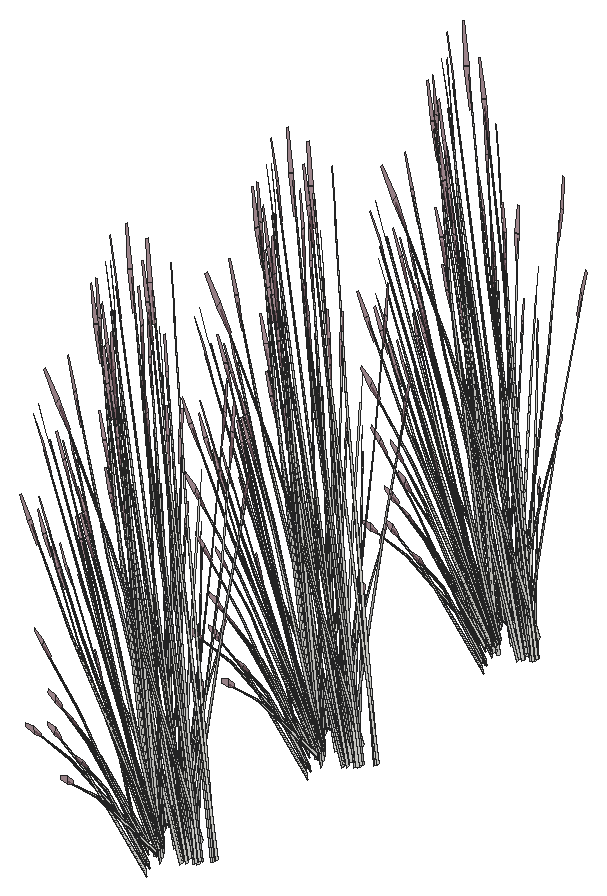
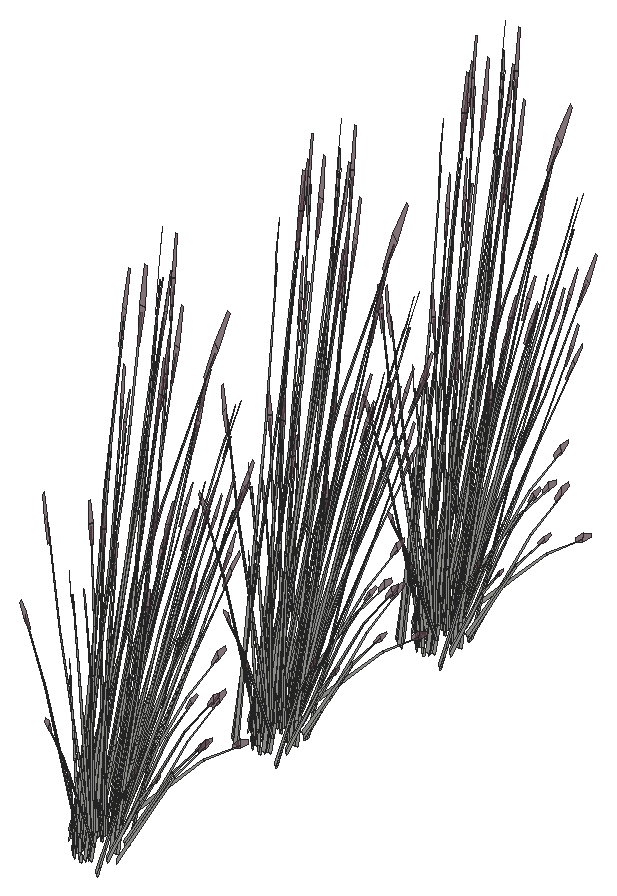
# SketchUp Ruby script. Lengths in inches.
U = 1.inch
M = Sketchup.active_model
def pt(a) = Geom::Point3d.new(a.map { |v| v * U })
def face(e, loops, mat)
  f = e.add_face(loops[0].map { |a| pt(a) })
  loops[1..].each { |l| e.add_face(l.map { |a| pt(a) }).erase! }
  f.material = f.back_material = mat if mat
  f
end
# faces: each face lists its corners as indices into pts; further lists are holes
def faces(e, pts, list, mat = nil) = list.each { |f| face(e, (f[0].is_a?(Array) ? f : [f]).map { |l| l.map { |i| pts[i] } }, mat) }
# xy, xz, yz: faces in a plane at the given z, y or x. An outline is a flat list of corners, or four numbers for a rectangle; further outlines are holes
def ring(l) = l.size == 4 ? [[l[0], l[1]], [l[2], l[1]], [l[2], l[3]], [l[0], l[3]]] : l.each_slice(2).to_a
def flat(e, list, mat, &to3) = list.each { |f| face(e, (f[0].is_a?(Array) ? f : [f]).map { |l| ring(l).map { |u, v| to3.(u, v) } }, mat) }
def xy(e, z, list, mat = nil) = flat(e, list, mat) { |x, y| [x, y, z] }
def xz(e, y, list, mat = nil) = flat(e, list, mat) { |x, z| [x, y, z] }
def yz(e, x, list, mat = nil) = flat(e, list, mat) { |y, z| [x, y, z] }
def lines(e, pts, list) = list.each { |a, b| e.add_line(pt(pts[a]), pt(pts[b])) }
# prism: a flat outline (further loops are holes) pulled along v
def prism(e, loops, v, mat = nil)
  f = face(e, loops, mat); d = Geom::Vector3d.new(v.map { |x| x * U })
  f.pushpull(f.normal.samedirection?(d) ? d.length : -d.length)
end
def box(e, o, s, mat = nil) = prism(e, [[o, [o[0] + s[0], o[1], o[2]], [o[0] + s[0], o[1] + s[1], o[2]], [o[0], o[1] + s[1], o[2]]]], [0, 0, s[2]], mat)
def at(x, y, z, deg = 0) = Geom::Transformation.translation(pt([x, y, z])) * Geom::Transformation.rotation(ORIGIN, Z_AXIS, deg.degrees)
def axes(o, x, y, z) = Geom::Transformation.new([*x, 0, *y, 0, *z, 0, *pt(o).to_a, 1])
def part(name) = M.definitions.add(name)
# library, detail: a bought-in or finely detailed component or shape, given as its bounding box
def library(name, o, s) = part(name).tap { |d| box(d.entities, o, s) }
def detail(e, o, s) = box(e.add_group.entities, o, s)
def put(e, d, t, mat = nil) = e.add_instance(d, t).tap { |i| i.material = mat if mat }
def group(e, t, mat = nil) = e.add_group.tap { |g| g.transformation = t; g.material = mat if mat }.entities
root = M.entities
M.materials.add("LightPink_Translucent").color = [144, 107, 117]
M.materials["LightPink_Translucent"].alpha = 0.75
c1 = part("blade")
p = [[2.15,0.21,22],[0,0.17,0],[0.09,0.45,0],[2.18,0.31,22],[2.29,0.31,22],[0.38,0.45,0],
  [2.48,0.24,33],[2.49,0.24,33],[2.48,0.22,33]]
faces(c1.entities,p,[[0,1,2,3],[4,5,2,3],[6,3,4,7],[8,0,3,6]])
c2 = part("seeds")
p = [[0.3,-0.1,1.38],[-0.01,-0.03,1.59],[-0.01,-0.03,0.03],[0.14,-0.07,-0.07],[0.29,-0.03,3],[0.15,0.01,3.11]]
faces(c2.entities,p,[[0,1,2,3],[1,0,4,5]],"LightPink_Translucent")
c3 = part("blade with seeds")
put(c3.entities,c1,at(0,0,0))
put(c3.entities,c2,axes([2.4,0.25,30.99],[1.5799,-0.05474,1.17369],[-0.12525,1.92788,0.29478],[-0.07173,-0.02425,1.56792]))
put(root,c3,axes([505.72,495.22,3.91],[-0.11621,-0.08567,1.74944],[-0.77555,0.05431,-0.27667],[-0.12378,-0.20491,0.14031]))
put(root,c3,axes([504.18,496,1.78],[-0.04601,0.19989,1.43002],[-0.67263,0.16733,-0.30754],[-0.15723,-0.25836,0.61141]))
put(root,c3,axes([504.93,494.94,3.9],[-0.01417,0.07324,1.77383],[-0.6991,0.2658,-0.16761],[-0.20573,-0.13587,0.31391]))
put(root,c3,axes([504.77,496.24,4.29],[0.84639,-0.15705,0.53763],[0.14689,0.61608,0.4433],[-0.19906,-0.18157,1.11249]))
put(root,c3,axes([503.95,495.68,1.96],[0.39634,0.21267,1.1486],[-0.57721,0.12784,0.84392],[-0.1235,-0.16344,0.25299]))
put(root,c3,axes([504.9,496.81,4.17],[-0.64788,-0.29534,-0.71045],[0.46044,-0.51755,0.08574],[-0.23473,-0.17635,1.00501]))
put(root,c3,axes([504.68,496.42,3.72],[-0.11735,-0.49217,-0.35414],[0.67083,-0.12996,0.4572],[-0.18018,-0.14104,0.87481]))
put(root,c3,axes([504.97,496.37,3.92],[0.34533,-0.38816,0.0643],[0.49176,0.22599,0.50621],[-0.15898,-0.12445,0.77189]))
put(root,c3,axes([503.63,496.32,0.6875],[-0.0736,0.08049,1.76342],[-0.74378,0.17355,-0.26939],[-0.17968,-0.15788,0.30037]))
put(root,c3,axes([504.6,496.82,3.875],[-0.74975,0.14525,-0.51099],[-0.13115,-0.55007,-0.3958],[-0.20138,-0.15763,0.97773]))
put(root,c3,axes([505.125,496.33,4.62],[-0.50709,0.58578,-0.13619],[-0.73436,-0.33748,-0.75594],[-0.25527,-0.1655,1.14864]))
put(root,c3,axes([503.18,496.16,3.91],[-0.16348,-0.00431,1.74944],[-0.52047,0.43131,-0.27667],[-0.2777,-0.08813,0.14031]))
put(root,c3,axes([506.45,500.15,2.52],[0.65659,0.2464,1.51261],[-0.64324,0.53082,0.59816],[-0.28812,-0.31461,1.26806]))
put(root,c3,axes([505.08,496.82,4.24],[0.11735,0.49217,0.35414],[-0.67083,0.12996,-0.4572],[-0.18018,-0.14104,0.87481]))
put(root,c3,axes([503.02,498.45,1.21],[0,-0.61104,-0.49651],[0.85008,0,0],[0,-0.13917,1.57504]))
put(root,c3,axes([503.0625,497.14,4.29],[0.62747,-0.45094,0.53763],[0.54116,0.47889,0.4433],[-0.29439,-0.08318,1.11249]))
put(root,c3,axes([503.35,497.14,3.92],[0.03826,-0.46465,0.0643],[0.57772,0.01274,0.50621],[-0.2213,-0.04862,0.77189]))
put(root,c3,axes([503.125,497.28,3.72],[-0.43232,-0.38257,-0.35414],[0.49364,-0.36215,0.4572],[-0.25081,-0.0551,0.87481]))
put(root,c3,axes([503.17,496.63,1.32],[-0.21918,0.49894,-0.03893],[-0.6746,-0.15348,-0.17649],[-0.10242,-0.08161,0.58215]))
put(root,c3,axes([502.81,498.91,1.57],[-0.95008,0,0],[0,-0.68292,-0.51607],[0,-0.15554,1.63711]))
put(root,c3,axes([503.54,498.73,1.52],[-0.70674,0.51372,0.30756],[-0.70717,-0.50832,-0.36492],[-0.02468,-0.14589,1.64885]))
put(root,c3,axes([505.46,499.8,1.63],[0.20138,-0.72405,-0.23429],[0.95485,0.12621,0.51271],[-0.16685,-0.09999,1.5644]))
put(root,c3,axes([503.74,497.48,4.24],[0.43232,0.38257,0.35414],[-0.49364,0.36215,-0.4572],[-0.25081,-0.0551,0.87481]))
put(root,c3,axes([502.09,498.2,1.96],[0.48508,-0.04372,1.1486],[-0.3077,0.38525,0.84392],[-0.23971,-0.05779,0.25299]))
put(root,c3,axes([503.62,497.24,4.23],[-0.04068,0.62141,-0.1216],[-0.77029,-0.01698,-0.67495],[-0.29667,-0.04317,1.02557]))
put(root,c3,axes([503.38,499.01,1.67],[0,0.61104,0.49651],[-0.85008,0,0],[0,-0.13917,1.57504]))
put(root,c3,axes([505.39,499.51,1.4],[-0.45644,-0.51287,-0.44739],[0.69137,-0.36116,0.21531],[-0.14771,-0.06346,1.43643]))
put(root,c3,axes([504.98,499.7,1.25],[-0.79037,-0.10018,-0.62353],[0.16679,-0.61794,-0.16365],[-0.23587,-0.07488,1.37633]))
put(root,c3,axes([502.51,498.55,3.93],[0.21466,-0.55714,0.48003],[0.70573,0.19051,0.3958],[-0.27753,0.03348,0.9933]))
put(root,c3,axes([502.46,498.4,3.92],[-0.27906,-0.41663,0.0643],[0.50888,-0.20393,0.50621],[-0.22432,0.04024,0.77189]))
put(root,c3,axes([504.14,500.64,1.22],[-0.17848,-0.53243,-0.30978],[0.70886,-0.15119,0.30978],[-0.1429,-0.0614,1.38974]))
put(root,c3,axes([503.94,500.87,1.21],[-0.7111,-0.30552,-0.49651],[0.42504,-0.54784,0],[-0.16196,-0.06958,1.57504]))
put(root,c3,axes([505.88,499.79,1.86],[-0.76714,0.40567,-0.29095],[-0.51013,-0.57321,-0.50002],[-0.18927,-0.05821,1.59708]))
put(root,c3,axes([505.81,499.97,1.81],[-0.14658,0.54532,0.1448],[-0.71613,-0.09466,-0.41347],[-0.13033,-0.05599,1.26744]))
put(root,c3,axes([503.03,498.56,4.24],[0.63144,0.17046,0.35414],[-0.18417,0.49731,-0.4572],[-0.25423,0.0456,0.87481]))
put(root,c3,axes([506.74,499.98,1.66],[-0.74193,-0.49181,-0.25192],[0.6243,-0.55226,0.5513],[-0.19979,0.05753,1.68216]))
put(root,c3,axes([504.79,500.92,1.67],[0.7111,0.30552,0.49651],[-0.42504,0.54784,0],[-0.16196,-0.06958,1.57504]))
put(root,c3,axes([502.76,498.39,4.23],[0.38229,0.5533,-0.1216],[-0.6785,0.2719,-0.67495],[-0.28593,0.073,1.02557]))
put(root,c3,axes([504.38,501.24,1.57],[-0.47504,0.61229,0],[-0.79476,-0.34146,-0.51607],[-0.18101,-0.07777,1.63711]))
put(root,c3,axes([506.36,499.875,1.4],[-0.82508,0.03772,-0.44739],[-0.07462,-0.62614,0.21531],[-0.14771,0.06346,1.43643]))
put(root,c3,axes([507.28,501.33,1.39],[-0.46912,-0.61443,-0.05142],[0.79476,-0.34146,0.51607],[-0.19584,0.0585,1.6363]))
put(root,c3,axes([502.68,499.9375,3.93],[-0.18844,-0.56237,0.48003],[0.73919,-0.0976,0.3958],[-0.21785,0.13226,0.9933]))
put(root,c3,axes([502.53,499.83,3.92],[-0.52161,-0.25698,0.0643],[0.30368,-0.36595,0.50621],[-0.16723,0.11831,0.77189]))
put(root,c3,axes([507.0625,501.25,1.22],[-0.70886,-0.15119,-0.30978],[0.17848,-0.53243,0.30978],[-0.1429,0.0614,1.38974]))
put(root,c3,axes([503.13,499.75,4.24],[0.66138,-0.08733,0.35414],[0.17464,0.49921,-0.4572],[-0.18953,0.13408,0.87481]))
put(root,c3,axes([501.4,501.24,1.96],[0.31665,-0.27694,1.1486],[0.12495,0.43841,0.84392],[-0.22883,0.0785,0.25299]))
put(root,c3,axes([502.59,500.05,3.72],[-0.66138,0.08733,-0.35414],[-0.17464,-0.49921,0.4572],[-0.18953,0.13408,0.87481]))
put(root,c3,axes([501.63,501.17,4.84],[0.67048,0.16311,-0.06488],[-0.20625,0.50201,-0.29416],[-0.10966,0.07622,0.97024]))
put(root,c3,axes([506.39,500.24,1.25],[-0.51177,0.45928,-0.62353],[-0.63575,-0.41646,-0.16365],[-0.20507,0.11457,1.37633]))
put(root,c3,axes([507.23,501.49,1.21],[-0.7111,0.30552,-0.49651],[-0.42504,-0.54784,0],[-0.16196,0.06958,1.57504]))
put(root,c3,axes([502.79,499.7,4.23],[0.70283,0.33692,-0.1216],[-0.40491,0.48793,-0.67495],[-0.19857,0.16961,1.02557]))
put(root,c3,axes([503.74,499.55,3.07],[0.18977,-0.18775,1.71376],[0.47917,0.50677,0.13857],[-0.32866,0.23079,0.73262]))
put(root,c3,axes([503.14,500.1,3.875],[0.19519,0.55794,-0.51099],[-0.73919,0.0976,-0.3958],[-0.21183,0.14986,0.97773]))
put(root,c3,axes([503.56,501.04,3.92],[-0.62439,-0.02847,0.0643],[0.01712,-0.42991,0.50621],[-0.06534,0.16468,0.77189]))
put(root,c3,axes([502.23,501.53,0.6875],[0.10192,0.06105,1.76342],[0.17281,0.56562,-0.26939],[-0.22588,0.12062,0.30037]))
put(root,c3,axes([503.76,501.08,3.93],[-0.54105,-0.41691,0.48003],[0.57458,-0.35956,0.3958],[-0.0998,0.1956,0.9933]))
put(root,c3,axes([503.59,500.02,3.07],[0.14147,-0.21002,1.71376],[0.59349,0.43464,0.13857],[-0.26773,0.27089,0.73262]))
put(root,c3,axes([503.76,501.2,3.72],[-0.5141,0.32171,-0.35414],[-0.48666,-0.36734,0.4572],[-0.07405,0.18664,0.87481]))
put(root,c3,axes([501.98,501.11,3.91],[-0.01889,0.12092,1.74944],[0.53598,0.42065,-0.27667],[-0.14032,0.19892,0.14031]))
put(root,c3,axes([504.08,502.45,1.96],[-0.01966,-0.36332,1.1486],[0.49135,0.25914,0.84392],[-0.09663,0.17317,0.25299]))
put(root,c3,axes([504.27,501.05,4.2],[0.54391,0.41056,-0.5672],[-0.57458,0.35956,-0.43934],[-0.08276,0.2086,1.08528]))
put(root,c3,axes([504.1,500.86,4.53],[-0.01977,0.56521,-0.7886],[-0.83252,-0.03796,0.09517],[-0.08786,0.23945,1.11556]))
put(root,c3,axes([501.92,502.35,3.9],[0.0862,-0.03689,1.77383],[0.71245,0.24539,-0.16761],[-0.01674,0.20431,0.31391]))
put(root,c3,axes([503.51,502.13,1.78],[0.23977,-0.09639,1.43002],[0.59198,0.29065,-0.30754],[-0.1762,0.25149,0.61141]))
put(root,c3,axes([503.82,501.66,2.56],[0.01669,-0.31544,1.54345],[0.75083,0.16661,0.21329],[-0.06506,0.33618,0.72882]))
put(root,c3,axes([504.63,518.62,3.07],[0.17368,0.19618,1.71376],[-0.80256,0.16516,0.13857],[-0.18139,-0.30799,0.73262]))
put(root,c3,axes([505.96,517.32,3.91],[-0.11621,-0.08567,1.74944],[-0.77555,0.05431,-0.27667],[-0.12378,-0.20491,0.14031]))
put(root,c3,axes([504.41,518.1,1.78],[-0.04601,0.19989,1.43002],[-0.67263,0.16733,-0.30754],[-0.15723,-0.25836,0.61141]))
put(root,c3,axes([505.16,517.04,3.9],[-0.01417,0.07324,1.77383],[-0.6991,0.2658,-0.16761],[-0.20573,-0.13587,0.31391]))
put(root,c3,axes([505.01,518.34,4.29],[0.84639,-0.15705,0.53763],[0.14689,0.61608,0.4433],[-0.19906,-0.18157,1.11249]))
put(root,c3,axes([504.18,517.78,1.96],[0.39634,0.21267,1.1486],[-0.57721,0.12784,0.84392],[-0.1235,-0.16344,0.25299]))
put(root,c3,axes([505.14,518.91,4.17],[-0.64788,-0.29534,-0.71045],[0.46044,-0.51755,0.08574],[-0.23473,-0.17635,1.00501]))
put(root,c3,axes([504.91,518.52,3.72],[-0.11735,-0.49217,-0.35414],[0.67083,-0.12996,0.4572],[-0.18018,-0.14104,0.87481]))
put(root,c3,axes([505.2,518.47,3.92],[0.34533,-0.38816,0.0643],[0.49176,0.22599,0.50621],[-0.15898,-0.12445,0.77189]))
put(root,c3,axes([503.87,518.42,0.6875],[-0.0736,0.08049,1.76342],[-0.74378,0.17355,-0.26939],[-0.17968,-0.15788,0.30037]))
put(root,c3,axes([504.83,518.92,3.875],[-0.74975,0.14525,-0.51099],[-0.13115,-0.55007,-0.3958],[-0.20138,-0.15763,0.97773]))
put(root,c3,axes([505.36,518.43,4.62],[-0.50709,0.58578,-0.13619],[-0.73436,-0.33748,-0.75594],[-0.25527,-0.1655,1.14864]))
put(root,c3,axes([503.41,518.26,3.91],[-0.16348,-0.00431,1.74944],[-0.52047,0.43131,-0.27667],[-0.2777,-0.08813,0.14031]))
put(root,c3,axes([506.6875,522.25,2.52],[0.65659,0.2464,1.51261],[-0.64324,0.53082,0.59816],[-0.28812,-0.31461,1.26806]))
put(root,c3,axes([505.31,518.92,4.24],[0.11735,0.49217,0.35414],[-0.67083,0.12996,-0.4572],[-0.18018,-0.14104,0.87481]))
put(root,c3,axes([503.25,520.54,1.21],[0,-0.61104,-0.49651],[0.85008,0,0],[0,-0.13917,1.57504]))
put(root,c3,axes([503.29,519.24,4.29],[0.62747,-0.45094,0.53763],[0.54116,0.47889,0.4433],[-0.29439,-0.08318,1.11249]))
put(root,c3,axes([503.58,519.23,3.92],[0.03826,-0.46465,0.0643],[0.57772,0.01274,0.50621],[-0.2213,-0.04862,0.77189]))
put(root,c3,axes([503.36,519.38,3.72],[-0.43232,-0.38257,-0.35414],[0.49364,-0.36215,0.4572],[-0.25081,-0.0551,0.87481]))
put(root,c3,axes([503.4,518.73,1.32],[-0.21918,0.49894,-0.03893],[-0.6746,-0.15348,-0.17649],[-0.10242,-0.08161,0.58215]))
put(root,c3,axes([503.04,521.01,1.57],[-0.95008,0,0],[0,-0.68292,-0.51607],[0,-0.15554,1.63711]))
put(root,c3,axes([503.78,520.83,1.52],[-0.70674,0.51372,0.30756],[-0.70717,-0.50832,-0.36492],[-0.02468,-0.14589,1.64885]))
put(root,c3,axes([502.79,518.63,3.9],[0.05633,0.06098,1.77383],[-0.27155,0.54815,-0.16761],[-0.27501,0.00397,0.31391]))
put(root,c3,axes([505.69,521.9,1.63],[0.20138,-0.72405,-0.23429],[0.95485,0.12621,0.51271],[-0.16685,-0.09999,1.5644]))
put(root,c3,axes([503.97,519.58,4.24],[0.43232,0.38257,0.35414],[-0.49364,0.36215,-0.4572],[-0.25081,-0.0551,0.87481]))
put(root,c3,axes([502.32,520.3,1.96],[0.48508,-0.04372,1.1486],[-0.3077,0.38525,0.84392],[-0.23971,-0.05779,0.25299]))
put(root,c3,axes([503.85,519.34,4.23],[-0.04068,0.62141,-0.1216],[-0.77029,-0.01698,-0.67495],[-0.29667,-0.04317,1.02557]))
put(root,c3,axes([503.62,521.11,1.67],[0,0.61104,0.49651],[-0.85008,0,0],[0,-0.13917,1.57504]))
put(root,c3,axes([505.625,521.6,1.4],[-0.45644,-0.51287,-0.44739],[0.69137,-0.36116,0.21531],[-0.14771,-0.06346,1.43643]))
put(root,c3,axes([505.22,521.8,1.25],[-0.79037,-0.10018,-0.62353],[0.16679,-0.61794,-0.16365],[-0.23587,-0.07488,1.37633]))
put(root,c3,axes([502.74,520.65,3.93],[0.21466,-0.55714,0.48003],[0.70573,0.19051,0.3958],[-0.27753,0.03348,0.9933]))
put(root,c3,axes([502.6875,520.5,3.92],[-0.27906,-0.41663,0.0643],[0.50888,-0.20393,0.50621],[-0.22432,0.04024,0.77189]))
put(root,c3,axes([504.375,522.74,1.22],[-0.17848,-0.53243,-0.30978],[0.70886,-0.15119,0.30978],[-0.1429,-0.0614,1.38974]))
put(root,c3,axes([504.18,522.97,1.21],[-0.7111,-0.30552,-0.49651],[0.42504,-0.54784,0],[-0.16196,-0.06958,1.57504]))
put(root,c3,axes([506.11,521.89,1.86],[-0.76714,0.40567,-0.29095],[-0.51013,-0.57321,-0.50002],[-0.18927,-0.05821,1.59708]))
put(root,c3,axes([506.04,522.07,1.81],[-0.14658,0.54532,0.1448],[-0.71613,-0.09466,-0.41347],[-0.13033,-0.05599,1.26744]))
put(root,c3,axes([503.26,520.65,4.24],[0.63144,0.17046,0.35414],[-0.18417,0.49731,-0.4572],[-0.25423,0.0456,0.87481]))
put(root,c3,axes([506.97,522.08,1.66],[-0.74193,-0.49181,-0.25192],[0.6243,-0.55226,0.5513],[-0.19979,0.05753,1.68216]))
put(root,c3,axes([505.02,523.02,1.67],[0.7111,0.30552,0.49651],[-0.42504,0.54784,0],[-0.16196,-0.06958,1.57504]))
put(root,c3,axes([503,520.49,4.23],[0.38229,0.5533,-0.1216],[-0.6785,0.2719,-0.67495],[-0.28593,0.073,1.02557]))
put(root,c3,axes([504.61,523.34,1.57],[-0.47504,0.61229,0],[-0.79476,-0.34146,-0.51607],[-0.18101,-0.07777,1.63711]))
put(root,c3,axes([506.6,521.97,1.4],[-0.82508,0.03772,-0.44739],[-0.07462,-0.62614,0.21531],[-0.14771,0.06346,1.43643]))
put(root,c3,axes([507.51,523.42,1.39],[-0.46912,-0.61443,-0.05142],[0.79476,-0.34146,0.51607],[-0.19584,0.0585,1.6363]))
put(root,c3,axes([502.91,522.03,3.93],[-0.18844,-0.56237,0.48003],[0.73919,-0.0976,0.3958],[-0.21785,0.13226,0.9933]))
put(root,c3,axes([502.77,521.93,3.92],[-0.52161,-0.25698,0.0643],[0.30368,-0.36595,0.50621],[-0.16723,0.11831,0.77189]))
put(root,c3,axes([503.37,521.85,4.24],[0.66138,-0.08733,0.35414],[0.17464,0.49921,-0.4572],[-0.18953,0.13408,0.87481]))
put(root,c3,axes([501.63,523.34,1.96],[0.31665,-0.27694,1.1486],[0.12495,0.43841,0.84392],[-0.22883,0.0785,0.25299]))
put(root,c3,axes([502.83,522.14,3.72],[-0.66138,0.08733,-0.35414],[-0.17464,-0.49921,0.4572],[-0.18953,0.13408,0.87481]))
put(root,c3,axes([501.87,523.26,4.84],[0.67048,0.16311,-0.06488],[-0.20625,0.50201,-0.29416],[-0.10966,0.07622,0.97024]))
put(root,c3,axes([506.62,522.33,1.25],[-0.51177,0.45928,-0.62353],[-0.63575,-0.41646,-0.16365],[-0.20507,0.11457,1.37633]))
put(root,c3,axes([507.46,523.59,1.21],[-0.7111,0.30552,-0.49651],[-0.42504,-0.54784,0],[-0.16196,0.06958,1.57504]))
put(root,c3,axes([503.02,521.8,4.23],[0.70283,0.33692,-0.1216],[-0.40491,0.48793,-0.67495],[-0.19857,0.16961,1.02557]))
put(root,c3,axes([503.97,521.65,3.07],[0.18977,-0.18775,1.71376],[0.47917,0.50677,0.13857],[-0.32866,0.23079,0.73262]))
put(root,c3,axes([503.37,522.2,3.875],[0.19519,0.55794,-0.51099],[-0.73919,0.0976,-0.3958],[-0.21183,0.14986,0.97773]))
put(root,c3,axes([503.79,523.13,3.92],[-0.62439,-0.02847,0.0643],[0.01712,-0.42991,0.50621],[-0.06534,0.16468,0.77189]))
put(root,c3,axes([502.47,523.625,0.6875],[0.10192,0.06105,1.76342],[0.17281,0.56562,-0.26939],[-0.22588,0.12062,0.30037]))
put(root,c3,axes([503.99,523.17,3.93],[-0.54105,-0.41691,0.48003],[0.57458,-0.35956,0.3958],[-0.0998,0.1956,0.9933]))
put(root,c3,axes([503.83,522.11,3.07],[0.14147,-0.21002,1.71376],[0.59349,0.43464,0.13857],[-0.26773,0.27089,0.73262]))
put(root,c3,axes([503.99,523.3,3.72],[-0.5141,0.32171,-0.35414],[-0.48666,-0.36734,0.4572],[-0.07405,0.18664,0.87481]))
put(root,c3,axes([502.22,523.2,3.91],[-0.01889,0.12092,1.74944],[0.53598,0.42065,-0.27667],[-0.14032,0.19892,0.14031]))
put(root,c3,axes([504.32,524.55,1.96],[-0.01966,-0.36332,1.1486],[0.49135,0.25914,0.84392],[-0.09663,0.17317,0.25299]))
put(root,c3,axes([504.33,522.96,4.53],[-0.01977,0.56521,-0.7886],[-0.83252,-0.03796,0.09517],[-0.08786,0.23945,1.11556]))
put(root,c3,axes([502.16,524.44,3.9],[0.0862,-0.03689,1.77383],[0.71245,0.24539,-0.16761],[-0.01674,0.20431,0.31391]))
put(root,c3,axes([503.75,524.23,1.78],[0.23977,-0.09639,1.43002],[0.59198,0.29065,-0.30754],[-0.1762,0.25149,0.61141]))
put(root,c3,axes([504.06,523.75,2.56],[0.01669,-0.31544,1.54345],[0.75083,0.16661,0.21329],[-0.06506,0.33618,0.72882]))
put(root,c3,axes([504.76,542.87,3.07],[0.17368,0.19618,1.71376],[-0.80256,0.16516,0.13857],[-0.18139,-0.30799,0.73262]))
put(root,c3,axes([504.54,542.35,1.78],[-0.04601,0.19989,1.43002],[-0.67263,0.16733,-0.30754],[-0.15723,-0.25836,0.61141]))
put(root,c3,axes([505.29,541.29,3.9],[-0.01417,0.07324,1.77383],[-0.6991,0.2658,-0.16761],[-0.20573,-0.13587,0.31391]))
put(root,c3,axes([505.14,542.59,4.29],[0.84639,-0.15705,0.53763],[0.14689,0.61608,0.4433],[-0.19906,-0.18157,1.11249]))
put(root,c3,axes([504.3125,542.03,1.96],[0.39634,0.21267,1.1486],[-0.57721,0.12784,0.84392],[-0.1235,-0.16344,0.25299]))
put(root,c3,axes([505.27,543.16,4.17],[-0.64788,-0.29534,-0.71045],[0.46044,-0.51755,0.08574],[-0.23473,-0.17635,1.00501]))
put(root,c3,axes([505.04,542.77,3.72],[-0.11735,-0.49217,-0.35414],[0.67083,-0.12996,0.4572],[-0.18018,-0.14104,0.87481]))
put(root,c3,axes([505.33,542.72,3.92],[0.34533,-0.38816,0.0643],[0.49176,0.22599,0.50621],[-0.15898,-0.12445,0.77189]))
put(root,c3,axes([504,542.67,0.6875],[-0.0736,0.08049,1.76342],[-0.74378,0.17355,-0.26939],[-0.17968,-0.15788,0.30037]))
put(root,c3,axes([504.96,543.17,3.875],[-0.74975,0.14525,-0.51099],[-0.13115,-0.55007,-0.3958],[-0.20138,-0.15763,0.97773]))
put(root,c3,axes([505.49,542.68,4.62],[-0.50709,0.58578,-0.13619],[-0.73436,-0.33748,-0.75594],[-0.25527,-0.1655,1.14864]))
put(root,c3,axes([503.54,542.51,3.91],[-0.16348,-0.00431,1.74944],[-0.52047,0.43131,-0.27667],[-0.2777,-0.08813,0.14031]))
put(root,c3,axes([506.82,546.5,2.52],[0.65659,0.2464,1.51261],[-0.64324,0.53082,0.59816],[-0.28812,-0.31461,1.26806]))
put(root,c3,axes([505.44,543.17,4.24],[0.11735,0.49217,0.35414],[-0.67083,0.12996,-0.4572],[-0.18018,-0.14104,0.87481]))
put(root,c3,axes([503.42,543.49,4.29],[0.62747,-0.45094,0.53763],[0.54116,0.47889,0.4433],[-0.29439,-0.08318,1.11249]))
put(root,c3,axes([503.71,543.49,3.92],[0.03826,-0.46465,0.0643],[0.57772,0.01274,0.50621],[-0.2213,-0.04862,0.77189]))
put(root,c3,axes([503.49,543.63,3.72],[-0.43232,-0.38257,-0.35414],[0.49364,-0.36215,0.4572],[-0.25081,-0.0551,0.87481]))
put(root,c3,axes([503.53,542.98,1.32],[-0.21918,0.49894,-0.03893],[-0.6746,-0.15348,-0.17649],[-0.10242,-0.08161,0.58215]))
put(root,c3,axes([503.17,545.26,1.57],[-0.95008,0,0],[0,-0.68292,-0.51607],[0,-0.15554,1.63711]))
put(root,c3,axes([503.91,545.08,1.52],[-0.70674,0.51372,0.30756],[-0.70717,-0.50832,-0.36492],[-0.02468,-0.14589,1.64885]))
put(root,c3,axes([502.92,542.88,3.9],[0.05633,0.06098,1.77383],[-0.27155,0.54815,-0.16761],[-0.27501,0.00397,0.31391]))
put(root,c3,axes([505.82,546.15,1.63],[0.20138,-0.72405,-0.23429],[0.95485,0.12621,0.51271],[-0.16685,-0.09999,1.5644]))
put(root,c3,axes([503.69,544.01,3.875],[-0.55171,0.40476,-0.51099],[-0.48318,-0.42758,-0.3958],[-0.28031,-0.06159,0.97773]))
put(root,c3,axes([504.1,543.83,4.24],[0.43232,0.38257,0.35414],[-0.49364,0.36215,-0.4572],[-0.25081,-0.0551,0.87481]))
put(root,c3,axes([502.45,544.55,1.96],[0.48508,-0.04372,1.1486],[-0.3077,0.38525,0.84392],[-0.23971,-0.05779,0.25299]))
put(root,c3,axes([503.98,543.59,4.23],[-0.04068,0.62141,-0.1216],[-0.77029,-0.01698,-0.67495],[-0.29667,-0.04317,1.02557]))
put(root,c3,axes([505.76,545.86,1.4],[-0.45644,-0.51287,-0.44739],[0.69137,-0.36116,0.21531],[-0.14771,-0.06346,1.43643]))
put(root,c3,axes([505.35,546.05,1.25],[-0.79037,-0.10018,-0.62353],[0.16679,-0.61794,-0.16365],[-0.23587,-0.07488,1.37633]))
put(root,c3,axes([502.875,544.9,3.93],[0.21466,-0.55714,0.48003],[0.70573,0.19051,0.3958],[-0.27753,0.03348,0.9933]))
put(root,c3,axes([502.82,544.75,3.92],[-0.27906,-0.41663,0.0643],[0.50888,-0.20393,0.50621],[-0.22432,0.04024,0.77189]))
put(root,c3,axes([502.81,545.18,0.6875],[0.01927,0.0963,1.76342],[-0.38846,0.5029,-0.26939],[-0.27592,-0.02535,0.30037]))
put(root,c3,axes([504.51,546.99,1.22],[-0.17848,-0.53243,-0.30978],[0.70886,-0.15119,0.30978],[-0.1429,-0.0614,1.38974]))
put(root,c3,axes([504.31,547.22,1.21],[-0.7111,-0.30552,-0.49651],[0.42504,-0.54784,0],[-0.16196,-0.06958,1.57504]))
put(root,c3,axes([506.24,546.14,1.86],[-0.76714,0.40567,-0.29095],[-0.51013,-0.57321,-0.50002],[-0.18927,-0.05821,1.59708]))
put(root,c3,axes([506.17,546.32,1.81],[-0.14658,0.54532,0.1448],[-0.71613,-0.09466,-0.41347],[-0.13033,-0.05599,1.26744]))
put(root,c3,axes([503.39,544.91,4.24],[0.63144,0.17046,0.35414],[-0.18417,0.49731,-0.4572],[-0.25423,0.0456,0.87481]))
put(root,c3,axes([507.1,546.33,1.66],[-0.74193,-0.49181,-0.25192],[0.6243,-0.55226,0.5513],[-0.19979,0.05753,1.68216]))
put(root,c3,axes([505.15,547.27,1.67],[0.7111,0.30552,0.49651],[-0.42504,0.54784,0],[-0.16196,-0.06958,1.57504]))
put(root,c3,axes([503.125,544.74,4.23],[0.38229,0.5533,-0.1216],[-0.6785,0.2719,-0.67495],[-0.28593,0.073,1.02557]))
put(root,c3,axes([504.74,547.59,1.57],[-0.47504,0.61229,0],[-0.79476,-0.34146,-0.51607],[-0.18101,-0.07777,1.63711]))
put(root,c3,axes([506.73,546.22,1.4],[-0.82508,0.03772,-0.44739],[-0.07462,-0.62614,0.21531],[-0.14771,0.06346,1.43643]))
put(root,c3,axes([503.04,546.29,3.93],[-0.18844,-0.56237,0.48003],[0.73919,-0.0976,0.3958],[-0.21785,0.13226,0.9933]))
put(root,c3,axes([502.9,546.18,3.92],[-0.52161,-0.25698,0.0643],[0.30368,-0.36595,0.50621],[-0.16723,0.11831,0.77189]))
put(root,c3,axes([503.5,546.1,4.24],[0.66138,-0.08733,0.35414],[0.17464,0.49921,-0.4572],[-0.18953,0.13408,0.87481]))
put(root,c3,axes([501.76,547.59,1.96],[0.31665,-0.27694,1.1486],[0.12495,0.43841,0.84392],[-0.22883,0.0785,0.25299]))
put(root,c3,axes([502.96,546.39,3.72],[-0.66138,0.08733,-0.35414],[-0.17464,-0.49921,0.4572],[-0.18953,0.13408,0.87481]))
put(root,c3,axes([502,547.52,4.84],[0.67048,0.16311,-0.06488],[-0.20625,0.50201,-0.29416],[-0.10966,0.07622,0.97024]))
put(root,c3,axes([506.75,546.59,1.25],[-0.51177,0.45928,-0.62353],[-0.63575,-0.41646,-0.16365],[-0.20507,0.11457,1.37633]))
put(root,c3,axes([503.15,546.05,4.23],[0.70283,0.33692,-0.1216],[-0.40491,0.48793,-0.67495],[-0.19857,0.16961,1.02557]))
put(root,c3,axes([504.1,545.9,3.07],[0.18977,-0.18775,1.71376],[0.47917,0.50677,0.13857],[-0.32866,0.23079,0.73262]))
put(root,c3,axes([503.5,546.45,3.875],[0.19519,0.55794,-0.51099],[-0.73919,0.0976,-0.3958],[-0.21183,0.14986,0.97773]))
put(root,c3,axes([503.92,547.39,3.92],[-0.62439,-0.02847,0.0643],[0.01712,-0.42991,0.50621],[-0.06534,0.16468,0.77189]))
put(root,c3,axes([502.6,547.875,0.6875],[0.10192,0.06105,1.76342],[0.17281,0.56562,-0.26939],[-0.22588,0.12062,0.30037]))
put(root,c3,axes([504.12,547.42,3.93],[-0.54105,-0.41691,0.48003],[0.57458,-0.35956,0.3958],[-0.0998,0.1956,0.9933]))
put(root,c3,axes([503.96,546.37,3.07],[0.14147,-0.21002,1.71376],[0.59349,0.43464,0.13857],[-0.26773,0.27089,0.73262]))
put(root,c3,axes([504.12,547.55,3.72],[-0.5141,0.32171,-0.35414],[-0.48666,-0.36734,0.4572],[-0.07405,0.18664,0.87481]))
put(root,c3,axes([502.35,547.45,3.91],[-0.01889,0.12092,1.74944],[0.53598,0.42065,-0.27667],[-0.14032,0.19892,0.14031]))
put(root,c3,axes([504.45,548.8,1.96],[-0.01966,-0.36332,1.1486],[0.49135,0.25914,0.84392],[-0.09663,0.17317,0.25299]))
put(root,c3,axes([504.46,547.21,4.53],[-0.01977,0.56521,-0.7886],[-0.83252,-0.03796,0.09517],[-0.08786,0.23945,1.11556]))
put(root,c3,axes([502.29,548.69,3.9],[0.0862,-0.03689,1.77383],[0.71245,0.24539,-0.16761],[-0.01674,0.20431,0.31391]))
put(root,c3,axes([503.875,548.48,1.78],[0.23977,-0.09639,1.43002],[0.59198,0.29065,-0.30754],[-0.1762,0.25149,0.61141]))
put(root,c3,axes([504.19,548.01,2.56],[0.01669,-0.31544,1.54345],[0.75083,0.16661,0.21329],[-0.06506,0.33618,0.72882]))
